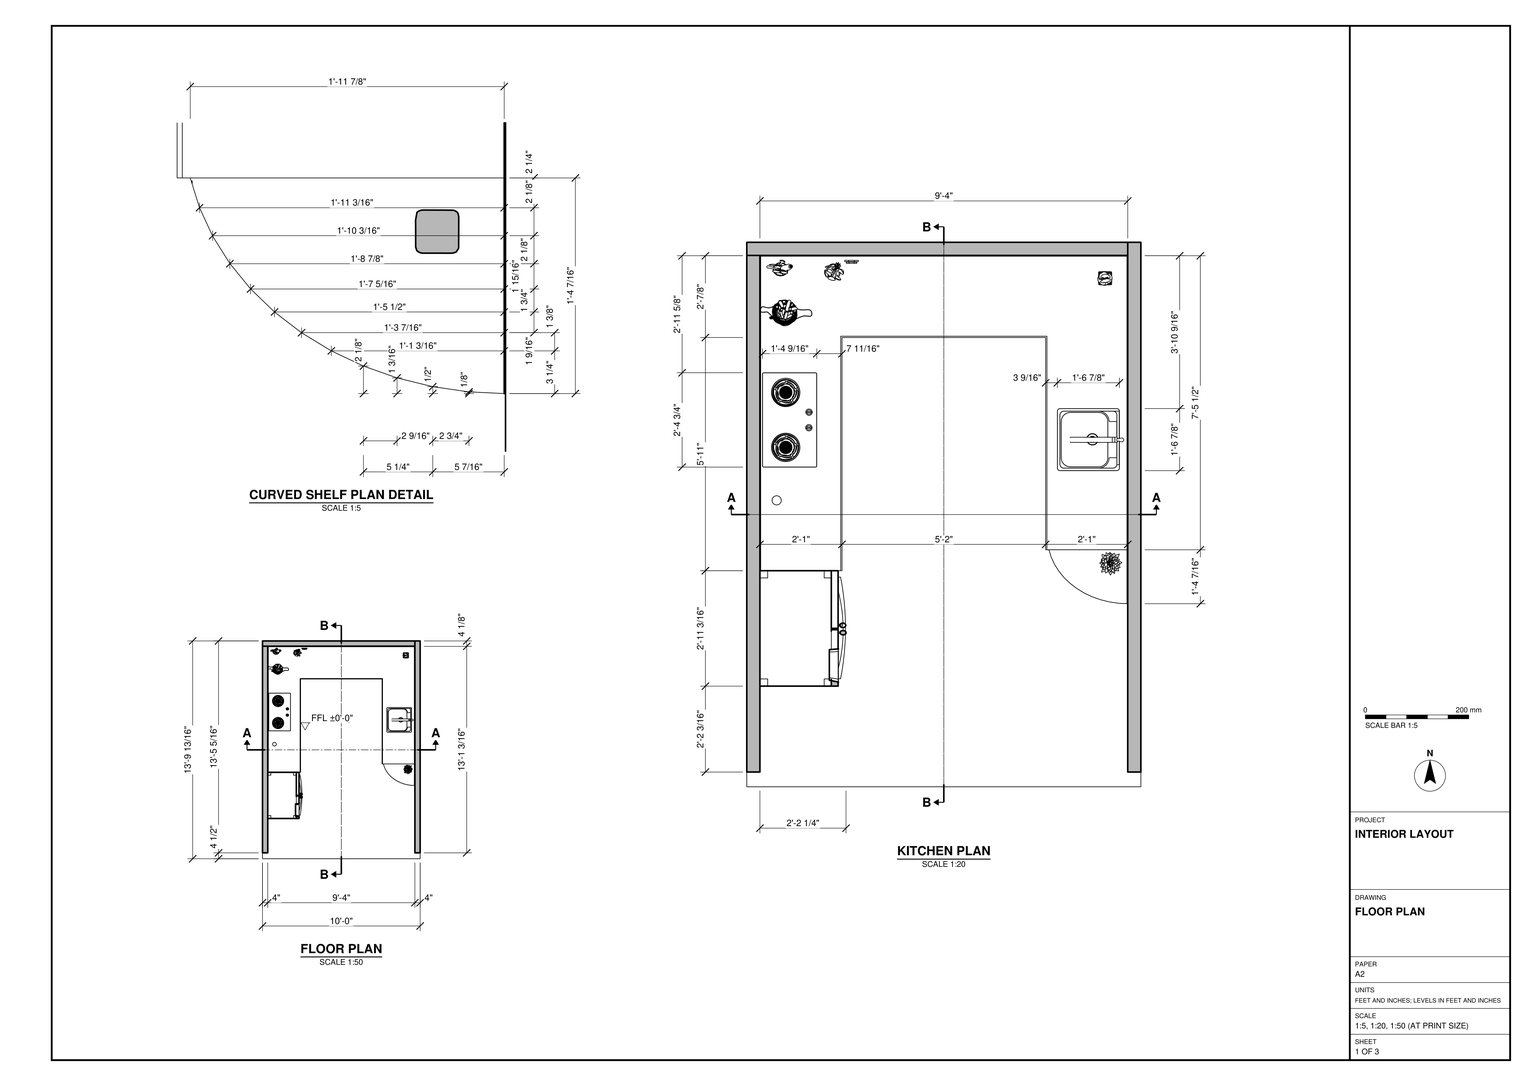
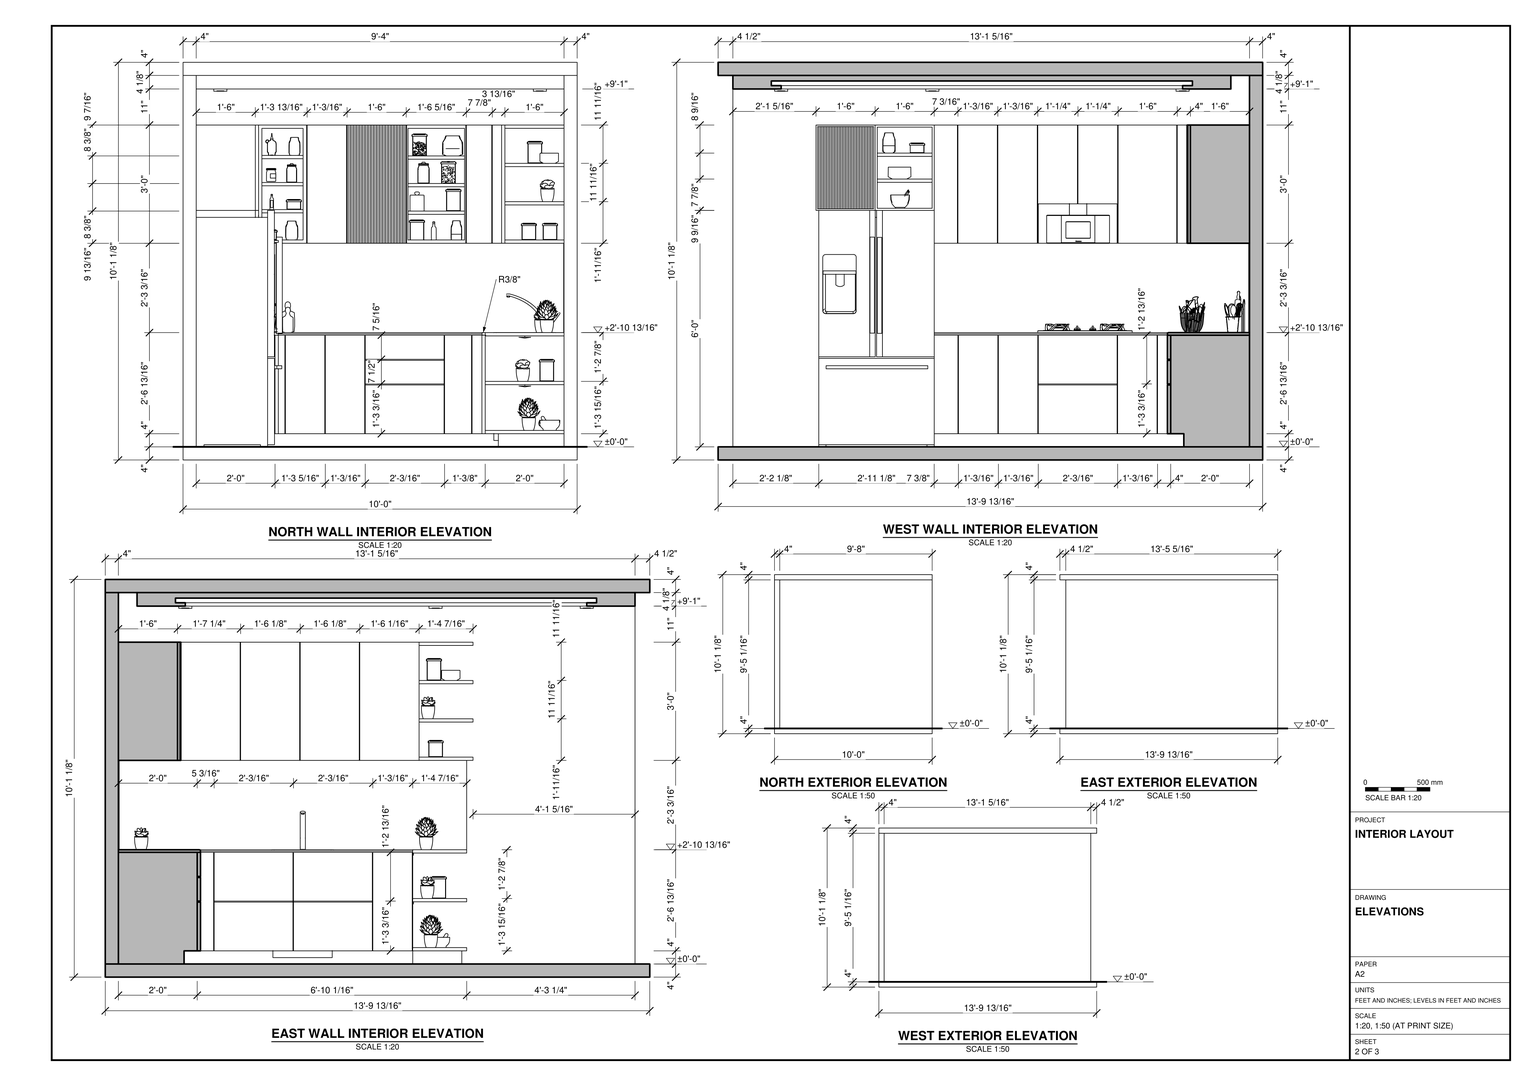
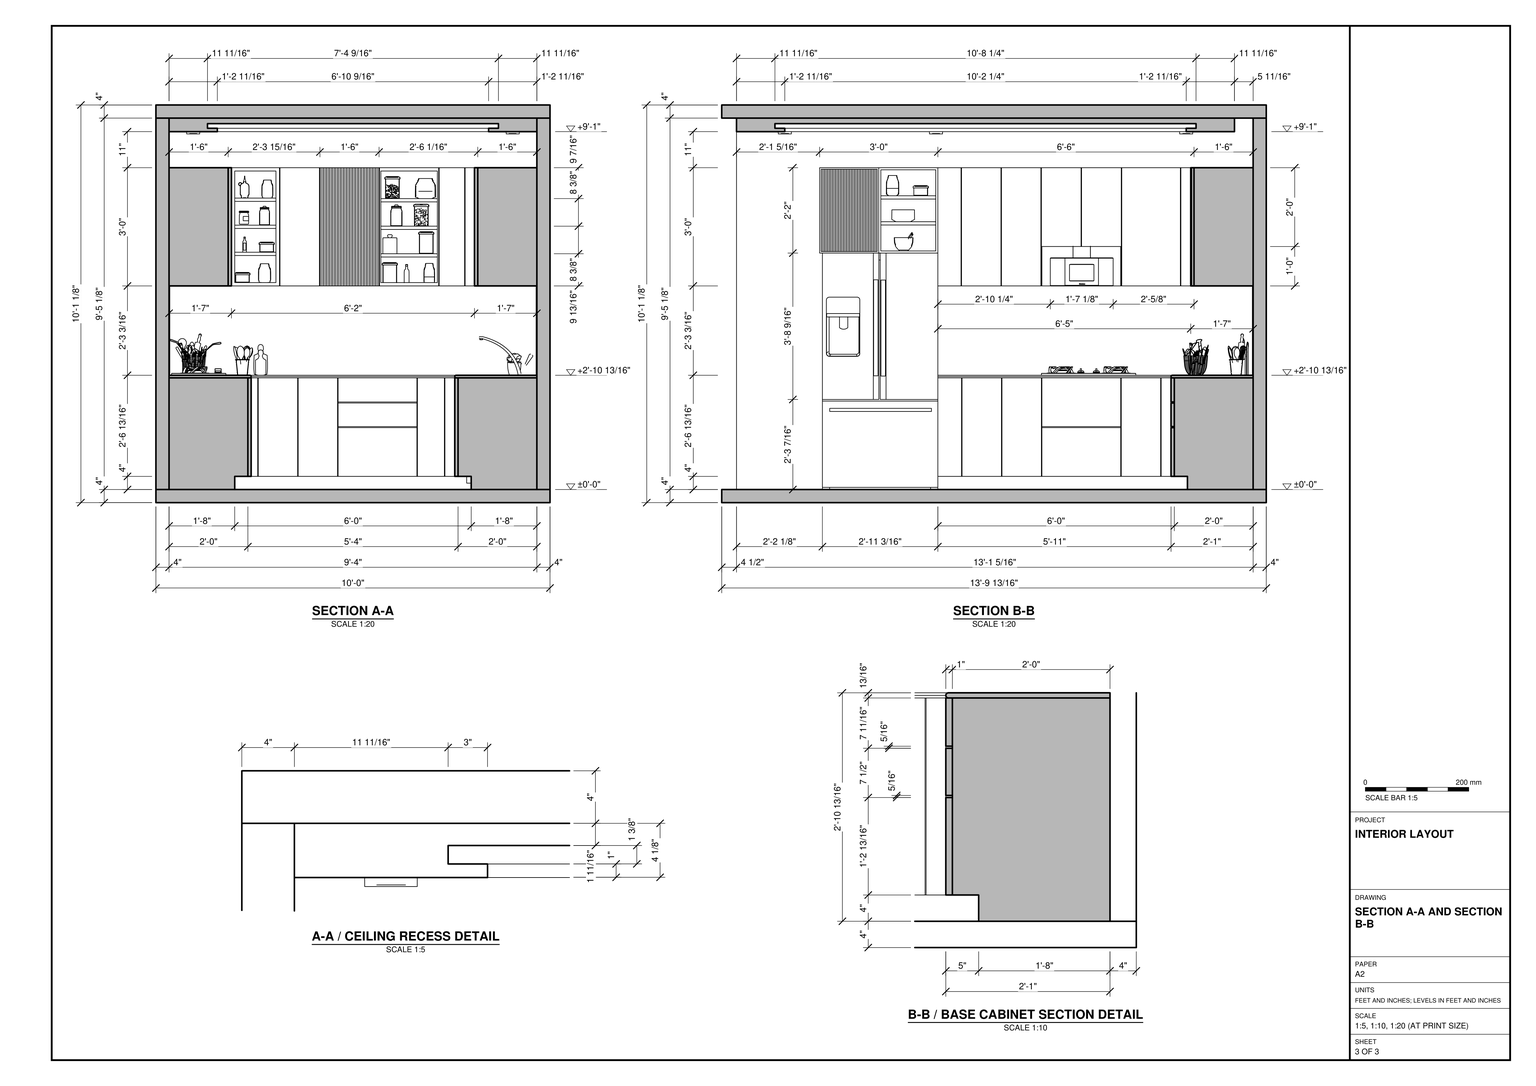
Build the kitchen interior in SketchUp from task_files/diagram_01.pdf. Work in feet and inches. Set the finished floor at ±0'-0". The overall model is 10'-0" wide, 13'-9 13/16" deep and 10'-1 1/8" high. Model the north wall and both side walls at the thicknesses shown, leaving the south end open. Include the floor slab, top slab and stepped ceiling recess shown in the sections.

Lay out the connected worktops along the west, north and east walls. Leave a 5'-2" aisle between the side runs. Place the cooktop on the west run, the refrigerator toward its open end, and the sink and tap on the east run. Follow the interior elevations for the recessed cabinet plinths, drawer banks, cupboard fronts and upper cabinets. Match the open shelf bays and vertically ribbed front on the north wall. Use the curved shelf plan detail to shape the exposed end of the east base run.

Appliances, lights, containers, utensils and plants may be any suitable library components. Keep the shell elements and each furniture or joinery piece in separate groups or components, and use components for repeated parts. Save one SketchUp model as output_files/u_shaped_kitchen_with_cabinetry_and_recessed_ceiling.skp.

# SketchUp Ruby script. Lengths in inches.
U = 1.inch
M = Sketchup.active_model
def pt(a) = Geom::Point3d.new(a.map { |v| v * U })
def face(e, loops, mat)
  f = e.add_face(loops[0].map { |a| pt(a) })
  loops[1..].each { |l| e.add_face(l.map { |a| pt(a) }).erase! }
  f.material = f.back_material = mat if mat
  f
end
# faces: each face lists its corners as indices into pts; further lists are holes
def faces(e, pts, list, mat = nil) = list.each { |f| face(e, (f[0].is_a?(Array) ? f : [f]).map { |l| l.map { |i| pts[i] } }, mat) }
# xy, xz, yz: faces in a plane at the given z, y or x. An outline is a flat list of corners, or four numbers for a rectangle; further outlines are holes
def ring(l) = l.size == 4 ? [[l[0], l[1]], [l[2], l[1]], [l[2], l[3]], [l[0], l[3]]] : l.each_slice(2).to_a
def flat(e, list, mat, &to3) = list.each { |f| face(e, (f[0].is_a?(Array) ? f : [f]).map { |l| ring(l).map { |u, v| to3.(u, v) } }, mat) }
def xy(e, z, list, mat = nil) = flat(e, list, mat) { |x, y| [x, y, z] }
def xz(e, y, list, mat = nil) = flat(e, list, mat) { |x, z| [x, y, z] }
def yz(e, x, list, mat = nil) = flat(e, list, mat) { |y, z| [x, y, z] }
def lines(e, pts, list) = list.each { |a, b| e.add_line(pt(pts[a]), pt(pts[b])) }
# prism: a flat outline (further loops are holes) pulled along v
def prism(e, loops, v, mat = nil)
  f = face(e, loops, mat); d = Geom::Vector3d.new(v.map { |x| x * U })
  f.pushpull(f.normal.samedirection?(d) ? d.length : -d.length)
end
def box(e, o, s, mat = nil) = prism(e, [[o, [o[0] + s[0], o[1], o[2]], [o[0] + s[0], o[1] + s[1], o[2]], [o[0], o[1] + s[1], o[2]]]], [0, 0, s[2]], mat)
def at(x, y, z, deg = 0) = Geom::Transformation.translation(pt([x, y, z])) * Geom::Transformation.rotation(ORIGIN, Z_AXIS, deg.degrees)
def axes(o, x, y, z) = Geom::Transformation.new([*x, 0, *y, 0, *z, 0, *pt(o).to_a, 1])
def part(name) = M.definitions.add(name)
# library, detail: a bought-in or finely detailed component or shape, given as its bounding box
def library(name, o, s) = part(name).tap { |d| box(d.entities, o, s) }
def detail(e, o, s) = box(e.add_group.entities, o, s)
def put(e, d, t, mat = nil) = e.add_instance(d, t).tap { |i| i.material = mat if mat }
def group(e, t, mat = nil) = e.add_group.tap { |g| g.transformation = t; g.material = mat if mat }.entities
root = M.entities
M.materials.add("Cl-3460 22.24cm").color = [255, 255, 255]
M.materials.add("Emissive").color = [255, 201, 138]
M.materials.add("Marble 005 36.41cm").color = [198, 200, 178]
M.materials.add("Marble Grey 23.82cm").color = [255, 255, 255]
M.materials.add("Marble Wood Grain 37.51cm").color = [255, 255, 255]
M.materials.add("VIdro preto coifa").color = [0, 0, 0]
M.materials["VIdro preto coifa"].alpha = 0.95
M.materials.add("Wood 021 27.52cm").color = [255, 255, 255]
M.materials.add("Wood Amboyan 13.2cm").color = [255, 255, 255]
M.materials.add("[Color M09]").color = [0, 0, 0]
M.materials.add("[Granite Dark Gray]").color = [69, 68, 68]
M.materials.add("[Stone Marble]").color = [143, 138, 136]
c1 = part("Shelf panel")
xy(c1.entities,0,[[-1.01,0,11.54,11.0625]],"Wood Amboyan 13.2cm")
xy(c1.entities,1,[[-1.01,0,11.54,11.0625]],"Wood Amboyan 13.2cm")
xz(c1.entities,0,[[-1.01,0,11.54,1]],"Wood Amboyan 13.2cm")
xz(c1.entities,11.0625,[[-1.01,0,11.54,1]])
yz(c1.entities,-1.01,[[0,0,11.0625,1]])
yz(c1.entities,11.54,[[0,0,11.0625,1]])
c2 = library("Fluted panel",[0,-0.1875,0],[18,0.1875,36])
c3 = part("Vertical slat")
box(c3.entities,[0,0,0],[1,0.39,25.06],"Cl-3460 22.24cm")
c4 = part("Group30\#1")
p = [[0,0,0],[0,0,-2.85],[-1.37,0,-2.85],[8.93,-0.3,0],[-8.93,-0.3,0],[8.93,0.3,0],
  [8.93,0,0],[-8.93,0.3,0],[1.37,0,-2.85],[-8.93,0,0],[0,0,-4.62]]
lines(c4.entities,p,[[0,1],[1,2],[3,4],[5,6],[7,5],[1,8],[9,0],[0,6],[8,10],[4,9],[6,3],[2,10],
  [9,7]])
c5 = part("Rectangle Light\#2")
put(c5.entities,c4,at(0,0,0))
c6 = part("Group32\#1")
p = [[0,0,0],[0,0,-2.83],[-1.375,0,-2.83],[8.95,-0.21,0],[-8.95,-0.21,0],[8.95,0.21,0],
  [8.95,0,0],[-8.95,0.21,0],[1.375,0,-2.83],[-8.95,0,0],[0,0,-4.58]]
lines(c6.entities,p,[[0,1],[1,2],[3,4],[5,6],[7,5],[1,8],[9,0],[0,6],[8,10],[4,9],[6,3],[2,10],
  [9,7]])
c7 = part("Rectangle Light\#3")
put(c7.entities,c6,at(0,0,0))
c8 = part("Group34\#1")
p = [[0,0,0],[0,0,-2.82],[-1.375,0,-2.82],[8.96,-0.18,0],[-8.96,-0.18,0],[8.96,0.18,0],
  [8.96,0,0],[-8.96,0.18,0],[1.375,0,-2.82],[-8.96,0,0],[0,0,-4.57]]
lines(c8.entities,p,[[0,1],[1,2],[3,4],[5,6],[7,5],[1,8],[9,0],[0,6],[8,10],[4,9],[6,3],[2,10],
  [9,7]])
c9 = part("Rectangle Light\#4")
put(c9.entities,c8,at(0,0,0))
c10 = part("Group36\#1")
p = [[0,0,0],[0,0,-2.96],[-1.32,0,-2.96],[8.6,-1,0],[-8.6,-1,0],[8.6,1,0],
  [8.6,0,0],[-8.6,1,0],[1.32,0,-2.96],[-8.6,0,0],[0,0,-4.8]]
lines(c10.entities,p,[[0,1],[1,2],[3,4],[5,6],[7,5],[1,8],[9,0],[0,6],[8,10],[4,9],[6,3],[2,10],
  [9,7]])
c11 = part("Rectangle Light\#5")
put(c11.entities,c10,at(0,0,0))
c12 = part("Group38\#1")
p = [[0,0,0],[0,0,-2.96],[-1.32,0,-2.96],[8.6,-0.97,0],[-8.6,-0.97,0],[8.6,0.97,0],
  [8.6,0,0],[-8.6,0.97,0],[1.32,0,-2.96],[-8.6,0,0],[0,0,-4.79]]
lines(c12.entities,p,[[0,1],[1,2],[3,4],[5,6],[7,5],[1,8],[9,0],[0,6],[8,10],[4,9],[6,3],[2,10],
  [9,7]])
c13 = part("Rectangle Light\#6")
put(c13.entities,c12,at(0,0,0))
c14 = part("Group40\#1")
p = [[0,0,0],[0,0,-3.02],[-1.32,0,-3.02],[8.6,-1.18,0],[-8.6,-1.18,0],[8.6,1.18,0],
  [8.6,0,0],[-8.6,1.18,0],[1.32,0,-3.02],[-8.6,0,0],[0,0,-4.89]]
lines(c14.entities,p,[[0,1],[1,2],[3,4],[5,6],[7,5],[1,8],[9,0],[0,6],[8,10],[4,9],[6,3],[2,10],
  [9,7]])
c15 = part("Rectangle Light\#7")
put(c15.entities,c14,at(0,0,0))
c16 = part("Group42\#1")
p = [[0,0,0],[0,0,-2.89],[-1.32,0,-2.89],[8.6,-0.76,0],[-8.6,-0.76,0],[8.6,0.76,0],
  [8.6,0,0],[-8.6,0.76,0],[1.32,0,-2.89],[-8.6,0,0],[0,0,-4.68]]
lines(c16.entities,p,[[0,1],[1,2],[3,4],[5,6],[7,5],[1,8],[9,0],[0,6],[8,10],[4,9],[6,3],[2,10],
  [9,7]])
c17 = part("Rectangle Light\#8")
put(c17.entities,c16,at(0,0,0))
c18 = part("Group44\#1")
p = [[0,0,0],[0,0,-2.23],[-0.96,0,-2.23],[6.28,-0.9375,0],[-6.28,-0.9375,0],[6.28,0.9375,0],
  [6.28,0,0],[-6.28,0.9375,0],[0.96,0,-2.23],[-6.28,0,0],[0,0,-3.61]]
lines(c18.entities,p,[[0,1],[1,2],[3,4],[5,6],[7,5],[1,8],[9,0],[0,6],[8,10],[4,9],[6,3],[2,10],
  [9,7]])
c19 = part("Rectangle Light\#9")
put(c19.entities,c18,at(0,0,0))
c20 = part("Group46\#1")
p = [[0,0,0],[0,0,-2.1],[-0.96,0,-2.1],[6.28,-0.54,0],[-6.28,-0.54,0],[6.28,0.54,0],
  [6.28,0,0],[-6.28,0.54,0],[0.96,0,-2.1],[-6.28,0,0],[0,0,-3.41]]
lines(c20.entities,p,[[0,1],[1,2],[3,4],[5,6],[7,5],[1,8],[9,0],[0,6],[8,10],[4,9],[6,3],[2,10],
  [9,7]])
c21 = part("Rectangle Light\#10")
put(c21.entities,c20,at(0,0,0))
c22 = part("Group48\#1")
p = [[0,0,0],[0,0,-2.11],[-0.96,0,-2.11],[6.28,-0.54,0],[-6.28,-0.54,0],[6.28,0.54,0],
  [6.28,0,0],[-6.28,0.54,0],[0.96,0,-2.11],[-6.28,0,0],[0,0,-3.41]]
lines(c22.entities,p,[[0,1],[1,2],[3,4],[5,6],[7,5],[1,8],[9,0],[0,6],[8,10],[4,9],[6,3],[2,10],
  [9,7]])
c23 = part("Rectangle Light\#11")
put(c23.entities,c22,at(0,0,0))
c24 = part("Group50\#1")
p = [[0,0,0],[0,0,-2.125],[-0.96,0,-2.125],[6.28,-0.6,0],[-6.28,-0.6,0],[6.28,0.6,0],
  [6.28,0,0],[-6.28,0.6,0],[0.96,0,-2.125],[-6.28,0,0],[0,0,-3.4375]]
lines(c24.entities,p,[[0,1],[1,2],[3,4],[5,6],[7,5],[1,8],[9,0],[0,6],[8,10],[4,9],[6,3],[2,10],
  [9,7]])
c25 = part("Rectangle Light\#12")
put(c25.entities,c24,at(0,0,0))
c26 = part("Group52\#1")
p = [[0,0,0],[0,0,-2.98],[-0.2,0,-2.98],[1.28,-8.36,0],[-1.28,-8.36,0],[1.28,8.36,0],
  [1.28,0,0],[-1.28,8.36,0],[0.2,0,-2.98],[-1.28,0,0],[0,0,-4.82]]
lines(c26.entities,p,[[0,1],[1,2],[3,4],[5,6],[7,5],[1,8],[9,0],[0,6],[8,10],[4,9],[6,3],[2,10],
  [9,7]])
c27 = part("Rectangle Light\#13")
put(c27.entities,c26,at(0,0,0))
c28 = part("Group54\#1")
p = [[0,0,0],[0,0,-2.93],[-0.17,0,-2.93],[1.13,-8.36,0],[-1.13,-8.36,0],[1.13,8.36,0],
  [1.13,0,0],[-1.13,8.36,0],[0.17,0,-2.93],[-1.13,0,0],[0,0,-4.75]]
lines(c28.entities,p,[[0,1],[1,2],[3,4],[5,6],[7,5],[1,8],[9,0],[0,6],[8,10],[4,9],[6,3],[2,10],
  [9,7]])
c29 = part("Rectangle Light\#14")
put(c29.entities,c28,at(0,0,0))
c30 = part("Group56\#1")
p = [[0,0,0],[0,0,-3.14],[-0.28,0,-3.14],[1.8125,-8.36,0],[-1.8125,-8.36,0],[1.8125,8.36,0],
  [1.8125,0,0],[-1.8125,8.36,0],[0.28,0,-3.14],[-1.8125,0,0],[0,0,-5.09]]
lines(c30.entities,p,[[0,1],[1,2],[3,4],[5,6],[7,5],[1,8],[9,0],[0,6],[8,10],[4,9],[6,3],[2,10],
  [9,7]])
c31 = part("Rectangle Light\#15")
put(c31.entities,c30,at(0,0,0))
c32 = part("Group58\#1")
p = [[0,0,0],[0,0,-17.95],[-8.6,0,-17.95],[56,-2.12,0],[-56,-2.12,0],[56,2.12,0],
  [56,0,0],[-56,2.12,0],[8.6,0,-17.95],[-56,0,0],[0,0,-29.06]]
lines(c32.entities,p,[[0,1],[1,2],[3,4],[5,6],[7,5],[1,8],[9,0],[0,6],[8,10],[4,9],[6,3],[2,10],
  [9,7]])
c33 = part("Rectangle Light\#16")
put(c33.entities,c32,at(0,0,0))
c34 = part("Group60\#1")
p = [[0,0,0],[0,0,-16.4],[-7.9,0,-16.4],[51.4,-1.7,0],[-51.4,-1.7,0],[51.4,1.7,0],
  [51.4,0,0],[-51.4,1.7,0],[7.9,0,-16.4],[-51.4,0,0],[0,0,-26.55]]
lines(c34.entities,p,[[0,1],[1,2],[3,4],[5,6],[7,5],[1,8],[9,0],[0,6],[8,10],[4,9],[6,3],[2,10],
  [9,7]])
c35 = part("Rectangle Light\#17")
put(c35.entities,c34,at(0,0,0))
c36 = library("double+fridge",[0,-4.28,0],[46.86,25.01,91.52])
c37 = library("GasStove_Black",[0,0,0],[28.74,16.54,2.72])
c38 = library("Potted Plant 50-23",[-3.4,-3.5,0],[6.8,7,9.93])
c39 = library("Potted Plant 50-24",[-2.18,-2.1,0],[4.36,4.2,6.7])
c40 = library("Kitchen Utensils 65-03",[-2.9,-2.77,0],[5.8,5.52,8.99])
c41 = library("Glass Vessel 001",[-1.95,-1.95,0.02],[3.9,3.9,7.26])
c42 = library("Decorative Jar 003",[-3.57,-2.61,0],[6.18,5.25,12.92])
c43 = library("Candy Jar 134 007 02",[-2.34,-2.34,0],[4.68,4.68,6.72])
c44 = library("Candy Jar 134 007 01",[-2.34,-2.34,0],[4.68,4.68,6.72])
c45 = library("Jar 83-03",[-2.15,-2.09,0],[4.3,4.18,5.88])
c46 = library("Sink and faucet",[-0.11,0,0],[20.3,18.9,21.51])
c47 = library("Kitchen Utensils 02 92-03",[-2.09,-0.47,0],[4.18,0.94,9.4])
c48 = library("Kitchen Utensils 01 92-03",[-3.91,-2.44,0],[7.79,4.85,12.66])
c49 = library("Group\#6",[0,0,0],[64,72,30])
c50 = part("Group\#49")
box(c50.entities,[0,0,0],[17.2,11.0625,1])
c51 = library("Group\#8",[0,0,0],[76,78,36])
c52 = part("Group\#20")
prism(c52.entities,[[[20,16.42,0],[20,0,0],[17.67,0.13,0],[15.37,0.53,0],[13.13,1.19,0],[10.98,2.1,0],[8.95,3.25,0],[7.0625,4.63,0],[5.35,6.21,0],[3.82,7.98,0],[2.51,9.91,0],[1.42,11.98,0],[0.59,14.16,0],[0,16.42,0]]],[0,0,1])
c53 = part("Group22\#1")
p = [[0,0,0],[0,0,-3.76],[-1.83,0,-3.76],[11.93,-0.24,0],[-11.93,-0.24,0],[11.93,0.24,0],
  [11.93,0,0],[-11.93,0.24,0],[1.83,0,-3.76],[-11.93,0,0],[0,0,-6.08]]
lines(c53.entities,p,[[0,1],[1,2],[3,4],[5,6],[7,5],[1,8],[9,0],[0,6],[8,10],[4,9],[6,3],[2,10],
  [9,7]])
c54 = part("Rectangle Light")
put(c54.entities,c53,at(0,0,0))
c55 = part("Group25\#1")
p = [[0,0,0],[0,0,-3.75],[-1.83,0,-3.75],[11.94,-0.21,0],[-11.94,-0.21,0],[11.94,0.21,0],
  [11.94,0,0],[-11.94,0.21,0],[1.83,0,-3.75],[-11.94,0,0],[0,0,-6.07]]
lines(c55.entities,p,[[0,1],[1,2],[3,4],[5,6],[7,5],[1,8],[9,0],[0,6],[8,10],[4,9],[6,3],[2,10],
  [9,7]])
c56 = part("Rectangle Light\#1")
put(c56.entities,c55,at(0,0,0))
c57 = library("Group\#12",[0,0,0],[112,96,0.79])
c58 = part("Group\#15")
box(c58.entities,[0,0,0],[13.375,16.72,1])
c59 = library("Agrupar\#3",[39.37,0,0],[35.43,16.85,31.3])
c60 = library("Group\#31",[0,0,0],[15.74,7.89,10.97])
c61 = library("Group\#32",[0,0,0],[4.68,4.68,6.72])
c62 = library("Group\#33",[0,0,0],[4.67,4.67,5.12])
c63 = library("Group\#34",[0,0,0],[4.68,4.68,3.1])
c64 = library("Group\#48",[0,0,0],[4.68,4.68,3.1])
c65 = library("Group\#35",[0,0,0],[4.68,4.68,6.72])
c66 = library("Group\#36",[0,0,0],[6.49,6.49,4.31])
c67 = library("Group\#37",[0,0,0],[2.64,2.64,11.07])
c68 = library("Group\#38",[0,0,0],[2.92,2.97,3.98])
c69 = library("Group\#39",[0,0,0],[2.6,2.61,11.08])
c70 = library("Group\#40",[0,0,0],[9.62,9.74,9.54])
c71 = library("Group\#41",[0,0,0],[7.36,7.36,7.28])
c72 = library("Group\#42",[0,0,0],[7.36,7.36,11.27])
c73 = library("Group\#43",[0,0,0],[5.95,5.95,9.65])
c74 = library("Group\#44",[0,0,0],[6.71,6.71,13.18])
c75 = library("Group\#47",[0,0,0],[5.95,5.95,9.65])
c76 = library("Recessed downlight",[0,0,0],[4,4,0.6875])
xy(root,38.79,[[115.9,55.76,116,161.71],[4,65.8125,4.1,161.71],[4,161.71,116,161.8125]])
xy(root,65.99,[[115.9,55.76,116,161.71],[4,161.71,116,161.8125]])
xy(root,66,[[4,65.8125,4.1,161.71]])
xz(root,55.76,[[115.9,38.79,116,65.99]],"[Stone Marble]")
xz(root,65.8125,[[4,38.79,4.1,66]],"[Stone Marble]")
xz(root,161.71,[[4,38.79,4.1,65.99],[115.9,38.79,116,65.99],[4,65.99,4.1,66]])
xz(root,161.71,[[4.1,38.79,115.9,65.99]],"Marble Grey 23.82cm")
xz(root,161.8125,[[4,38.79,116,65.99]])
yz(root,4,[[161.71,38.79,161.8125,65.99]])
yz(root,4.1,[[65.8125,38.79,161.71,66]],"[Stone Marble]")
yz(root,115.9,[[55.76,38.79,161.71,65.99]],"Marble Grey 23.82cm")
yz(root,116,[[161.71,38.79,161.8125,65.99]])
put(root,c1,at(25.01,143.8125,75.26))
put(root,c1,at(25.01,143.8125,83.5))
put(root,c1,at(25.01,143.8125,91.74))
put(root,c2,at(49.94,143,66))
put(root,c3,at(22,30.28,76.47))
put(root,c3,at(22,31.11,76.47))
put(root,c3,at(22,31.95,76.47))
put(root,c3,at(22,32.78,76.47))
put(root,c3,at(22,33.62,76.47))
put(root,c3,at(22,34.45,76.47))
put(root,c3,at(22,35.28,76.47))
put(root,c3,at(22,36.12,76.47))
put(root,c3,at(22,36.95,76.47))
put(root,c3,at(22,37.79,76.47))
put(root,c3,at(22,38.62,76.47))
put(root,c3,at(22,39.45,76.47))
put(root,c3,at(22,40.29,76.47))
put(root,c3,at(22,41.12,76.47))
put(root,c3,at(22,41.96,76.47))
put(root,c3,at(22,42.79,76.47))
put(root,c3,at(22,43.625,76.47))
put(root,c3,at(22,44.46,76.47))
put(root,c3,at(22,45.29,76.47))
put(root,c3,at(22,46.125,76.47))
put(root,c3,at(22,46.96,76.47))
put(root,c5,axes([107.07,69.95,100.99],[1,0,0],[0,1,0],[0,0,0.14]))
put(root,c7,axes([107.05,70.04,89.32],[1,0,0],[0,1,0],[0,0,0.23]))
put(root,c9,axes([107.04,70.07,77.66],[1,0,0],[0,1,0],[0,0,0.19]))
put(root,c11,axes([77.1,153.88,100.98],[1,0,0],[0,-1,0],[0,0,0.21]))
put(root,c13,axes([77.1,153.9,91.58],[1,0,0],[0,-1,0],[0,0,0.18]))
put(root,c15,axes([77.1,153.7,83.18],[1,0,0],[0,-1,0],[0,0,0.18]))
put(root,c17,axes([77.1,154.11,74.79],[1,0,0],[0,-1,0],[0,0,0.22]))
put(root,c19,axes([30.28,153.9375,100.98],[1,0,0],[0,-1,0],[0,0,0.2]))
put(root,c21,axes([30.28,154.34,91.73],[1,0,0],[0,-1,0],[0,0,0.25]))
put(root,c23,axes([30.28,154.33,83.49],[1,0,0],[0,-1,0],[0,0,0.17]))
put(root,c25,axes([30.28,154.27,75.25],[1,0,0],[0,-1,0],[0,0,0.19]))
put(root,c27,axes([9.9,56.8125,101.35],[1,0,0],[0,-1,0],[0,0,0.19]))
put(root,c29,axes([9.76,56.8125,92.44],[1,0,0],[0,1,0],[0,0,0.17]))
put(root,c31,axes([10.4375,56.8125,84.54],[1,0,0],[0,1,0],[0,0,0.17]))
put(root,c33,axes([60,159.69,65.99],[1,0,0],[0,-1,0],[0,0,0.11]))
put(root,c35,axes([114.3,106.17,66],[0,-1,0],[-1,0,0],[0,0,0.06059]))
put(root,c36,axes([25.74,30.66,4],[0,0.75,0],[-1.04843,0,0],[0,0,0.78669]))
put(root,c37,at(21.32,97.34,38.67,90))
put(root,c38,at(105.31,66.51,9))
put(root,c38,at(110.84,67.95,38.79))
put(root,c39,at(103.42,67.68,23.9375))
put(root,c39,at(109.0625,154.79,38.79))
put(root,c39,at(110.91,67.46,78.67))
put(root,c40,at(26.58,156.95,38.79))
put(root,c41,axes([73.22,146.92,84.2],[0.89,0,0],[0,0.89,0],[0,0,0.89]))
put(root,c41,axes([33.07,147.84,84.5],[0.79,0,0],[0,0.79,0],[0,0,0.79]))
put(root,c42,axes([27.02,145.43,92.75],[0.52,0,0],[0,0.52,0],[0,0,0.52]))
put(root,c43,at(72.01,151.24,92.59))
put(root,c44,at(80.8,147.93,84.19))
put(root,c45,at(71.25,148.48,75.75))
put(root,c46,at(114.77,115.17,29.05,180))
put(root,c47,at(31.89,159.85,38.79))
put(root,c48,at(10,157.99,38.79))
g1 = group(root,at(0,45.8125,0))
xy(g1,0,[[0,-45.8125,120,120]])
xy(g1,4,[[0,-45.8125,120,120]],"Marble 005 36.41cm")
xz(g1,-45.8125,[[0,0,120,4]])
xz(g1,120,[[0,0,120,4]])
yz(g1,0,[[-45.8125,0,120,4]])
yz(g1,120,[[-45.8125,0,120,4]])
g2 = group(root,at(116,45.8125,4))
box(g2,[0,-41.3125,0],[4,161.3125,113.1])
g3 = group(root,at(0,161.8125,4))
box(g3,[0,0,0],[116,4,113.1])
g4 = group(root,at(0,45.8125,4))
box(g4,[0,-41.3125,0],[4,157.3125,113.1])
g5 = group(root,at(4,65.8125,4))
xy(g5,0,[[0,0,0,96,112,96,112,6.37,92,6.37,92,76,20,76,20,0]])
xy(g5,1.9375,[[90.63,30.89,107.24,48.95]])
xy(g5,4,[[20,0,24,76],[88,6.37,92,72],[24,72,92,76]])
xy(g5,34,[[[0,0,24,0,24,72,88,72,88,6.37,112,6.37,112,96,0,96],[90.63,30.89,107.24,48.95]]])
xz(g5,0,[[0,0,20,0,20,4,24,4,24,34,0,34]])
xz(g5,6.37,[[92,0,112,0,112,34,88,34,88,4,92,4]])
xz(g5,30.89,[[90.63,1.9375,107.24,34]])
xz(g5,48.95,[[90.63,1.9375,107.24,34]])
xz(g5,72,[[24,4,88,34]])
xz(g5,76,[[20,0,92,4]],"Wood 021 27.52cm")
xz(g5,96,[[0,0,112,34]])
yz(g5,0,[[0,0,96,34]])
yz(g5,20,[[0,0,76,4]],"Wood 021 27.52cm")
yz(g5,24,[[0,4,72,34]])
yz(g5,88,[[6.37,4,72,34]])
yz(g5,90.63,[[30.89,1.9375,48.95,34]])
yz(g5,92,[[6.37,0,76,4]],"Wood 021 27.52cm")
yz(g5,107.24,[[30.89,1.9375,48.95,34]])
yz(g5,112,[[6.37,0,96,34]])
put(root,c49,at(28,65.8125,8),"Cl-3460 22.24cm")
g6 = group(root,at(4,65.8125,66))
xy(g6,0,[[0,0,18,31.69],[94,4.4375,94,78,18,78,18,55.69,0,55.69,0,96,112,96,112,4.4375]])
xy(g6,0.4,[[64.5,78,81.7,89.0625]])
xy(g6,1.01,[[20,78,32.55,89.0625]])
xy(g6,12,[[0,31.69,18,55.69]])
xy(g6,34.99,[[20,78,32.55,89.0625],[64.5,78,81.7,89.0625]])
xy(g6,36,[[0,0,18,0,18,78,94,78,94,4.4375,112,4.4375,112,96,0,96]])
xz(g6,0,[[0,0,18,36]])
xz(g6,4.4375,[[94,0,112,36]])
xz(g6,31.69,[[0,0,18,12]])
xz(g6,55.69,[[0,0,18,12]])
xz(g6,78,[[[18,0,94,36],[64.5,0.4,81.7,34.99],[20,1.01,32.55,34.99]]])
xz(g6,89.0625,[[64.5,0.4,81.7,34.99],[20,1.01,32.55,34.99]])
yz(g6,0,[[31.69,0,55.69,12]])
yz(g6,18,[[0,0,31.69,0,31.69,12,55.69,12,55.69,0,78,0,78,36,0,36]])
yz(g6,20,[[78,1.01,89.0625,34.99]])
yz(g6,32.55,[[78,1.01,89.0625,34.99]])
yz(g6,64.5,[[78,0.4,89.0625,34.99]])
yz(g6,81.7,[[78,0.4,89.0625,34.99]])
yz(g6,94,[[4.4375,0,78,36]])
yz(g6,112,[[4.4375,0,96,36]])
put(root,c50,at(68.5,143.8125,74.8),"Wood Amboyan 13.2cm")
put(root,c50,at(68.5,143.8125,83.19),"Wood Amboyan 13.2cm")
g7 = group(root,at(68.5,143.8125,91.59),"Wood Amboyan 13.2cm")
box(g7,[0,0,0],[17.2,11.0625,1])
put(root,c51,at(22,65.8125,66),"Cl-3460 22.24cm")
g8 = group(root,at(94.1,55.9,4),"[Color M09]")
prism(g8,[[[21.9,16.28,0],[21.9,1.34,0],[19.61,1.5625,0],[17.36,2,0],[15.17,2.65,0],[13.0625,3.51,0],[11.07,4.57,0],[9.21,5.8125,0],[7.51,7.23,0],[5.98,8.8,0],[4.64,10.51,0],[3.51,12.34,0],[2.59,14.27,0],[1.9,16.28,0]]],[0,0,4])
put(root,c52,axes([92,55.76,8],[1.2,0,0],[0,1,0],[0,0,1]),"[Granite Dark Gray]")
g9 = group(root,at(92,55.76,22.9375),"[Granite Dark Gray]")
xy(g9,0,[[24,0,21.2,0.13,18.44,0.53,15.75,1.19,13.18,2.1,10.74,3.25,8.47,4.63,6.41,6.21,4.58,7.98,3.01,9.91,1.71,11.98,0.7,14.16,0.15,15.94,24,15.94],[0.15,15.94,0,16.42,24,16.42,24,15.94]])
xy(g9,1,[[24,0,24,16.42,0,16.42,0.7,14.16,1.71,11.98,3.01,9.91,4.58,7.98,6.41,6.21,8.47,4.63,10.74,3.25,13.18,2.1,15.75,1.19,18.44,0.53,21.2,0.13]])
xz(g9,16.42,[[0,0,24,1]])
yz(g9,24,[[0,0,16.42,1]])
p = [[24,0,1],[21.2,0.13,1],[21.2,0.13,0],[24,0,0],[18.44,0.53,1],[18.44,0.53,0],
  [15.75,1.19,1],[15.75,1.19,0],[13.18,2.1,1],[13.18,2.1,0],[10.74,3.25,1],[10.74,3.25,0],
  [8.47,4.63,1],[8.47,4.63,0],[6.41,6.21,1],[6.41,6.21,0],[4.58,7.98,1],[4.58,7.98,0],
  [3.01,9.91,1],[3.01,9.91,0],[1.71,11.98,1],[1.71,11.98,0],[0.7,14.16,1],[0.7,14.16,0],
  [0,16.42,1],[0,16.42,0],[0.15,15.94,0],[24.15,15.94,0],[24,15.94,0]]
faces(g9,p,[[0,1,2,3],[1,4,5,2],[4,6,7,5],[6,8,9,7],[8,10,11,9],[10,12,13,11],[12,14,15,13],[14,16,17,15],
  [16,18,19,17],[18,20,21,19],[20,22,23,21],[22,24,25,26,23]])
lines(g9,p,[[27,28]])
put(g9,c54,axes([12.07,16.18,-0.01],[1,0,0],[0,1,0],[0,0,0.11]))
g10 = group(root,at(92,55.76,37.79),"[Granite Dark Gray]")
xy(g10,0,[[24,0,21.2,0.13,18.44,0.53,15.75,1.19,13.18,2.1,10.74,3.25,8.47,4.63,6.41,6.21,4.58,7.98,3.01,9.91,1.71,11.98,0.7,14.16,0.13,16,24,16],[0.13,16,0,16.42,24,16.42,24,16]])
xy(g10,1,[[24,0,24,16.42,0,16.42,0.7,14.16,1.71,11.98,3.01,9.91,4.58,7.98,6.41,6.21,8.47,4.63,10.74,3.25,13.18,2.1,15.75,1.19,18.44,0.53,21.2,0.13]])
xz(g10,16.42,[[0,0,24,1]])
yz(g10,24,[[0,0,16.42,1]])
p = [[24,0,1],[21.2,0.13,1],[21.2,0.13,0],[24,0,0],[18.44,0.53,1],[18.44,0.53,0],
  [15.75,1.19,1],[15.75,1.19,0],[13.18,2.1,1],[13.18,2.1,0],[10.74,3.25,1],[10.74,3.25,0],
  [8.47,4.63,1],[8.47,4.63,0],[6.41,6.21,1],[6.41,6.21,0],[4.58,7.98,1],[4.58,7.98,0],
  [3.01,9.91,1],[3.01,9.91,0],[1.71,11.98,1],[1.71,11.98,0],[0.7,14.16,1],[0.7,14.16,0],
  [0,16.42,1],[0,16.42,0],[0.13,16,0],[24.13,16,0],[24,16,0]]
faces(g10,p,[[0,1,2,3],[1,4,5,2],[4,6,7,5],[6,8,9,7],[8,10,11,9],[10,12,13,11],[12,14,15,13],[14,16,17,15],
  [16,18,19,17],[18,20,21,19],[20,22,23,21],[22,24,25,26,23]])
lines(g10,p,[[27,28]])
put(g10,c56,axes([12.06,16.21,-0.01],[1,0,0],[0,1,0],[0,0,0.11]))
g11 = group(root,at(98,53.83,101),"[Granite Dark Gray]")
xy(g11,0,[[18,0,15.9,0.13,13.83,0.53,11.82,1.19,9.88,2.1,8.05,3.25,6.36,4.63,4.8125,6.21,3.4375,7.98,2.26,9.91,1.28,11.98,0.53,14.16,0.14,15.81,18,15.81],[0.14,15.81,0,16.42,18,16.42,18,15.81]])
xy(g11,1,[[18,0,18,16.42,0,16.42,0.53,14.16,1.28,11.98,2.26,9.91,3.4375,7.98,4.8125,6.21,6.36,4.63,8.05,3.25,9.88,2.1,11.82,1.19,13.83,0.53,15.9,0.13]])
xz(g11,16.42,[[0,0,18,1]])
yz(g11,18,[[0,0,16.42,1]])
p = [[18,0,1],[15.9,0.13,1],[15.9,0.13,0],[18,0,0],[13.83,0.53,1],[13.83,0.53,0],
  [11.82,1.19,1],[11.82,1.19,0],[9.88,2.1,1],[9.88,2.1,0],[8.05,3.25,1],[8.05,3.25,0],
  [6.36,4.63,1],[6.36,4.63,0],[4.8125,6.21,1],[4.8125,6.21,0],[3.4375,7.98,1],[3.4375,7.98,0],
  [2.26,9.91,1],[2.26,9.91,0],[1.28,11.98,1],[1.28,11.98,0],[0.53,14.16,1],[0.53,14.16,0],
  [0,16.42,1],[0,16.42,0],[0.14,15.81,0],[18.14,15.81,0],[18,15.81,0]]
faces(g11,p,[[0,1,2,3],[1,4,5,2],[4,6,7,5],[6,8,9,7],[8,10,11,9],[10,12,13,11],[12,14,15,13],[14,16,17,15],
  [16,18,19,17],[18,20,21,19],[20,22,23,21],[22,24,25,26,23]])
lines(g11,p,[[27,28]])
g12 = group(root,at(98,53.83,89.33),"[Granite Dark Gray]")
xy(g12,0,[[18,0,15.9,0.13,13.83,0.53,11.82,1.19,9.88,2.1,8.05,3.25,6.36,4.63,4.8125,6.21,3.4375,7.98,2.26,9.91,1.28,11.98,0.53,14.16,0.1,15.99,18,15.99],[0.1,15.99,0,16.42,18,16.42,18,15.99]])
xy(g12,1,[[18,0,18,16.42,0,16.42,0.53,14.16,1.28,11.98,2.26,9.91,3.4375,7.98,4.8125,6.21,6.36,4.63,8.05,3.25,9.88,2.1,11.82,1.19,13.83,0.53,15.9,0.13]])
xz(g12,16.42,[[0,0,18,1]])
yz(g12,18,[[0,0,16.42,1]])
p = [[18,0,1],[15.9,0.13,1],[15.9,0.13,0],[18,0,0],[13.83,0.53,1],[13.83,0.53,0],
  [11.82,1.19,1],[11.82,1.19,0],[9.88,2.1,1],[9.88,2.1,0],[8.05,3.25,1],[8.05,3.25,0],
  [6.36,4.63,1],[6.36,4.63,0],[4.8125,6.21,1],[4.8125,6.21,0],[3.4375,7.98,1],[3.4375,7.98,0],
  [2.26,9.91,1],[2.26,9.91,0],[1.28,11.98,1],[1.28,11.98,0],[0.53,14.16,1],[0.53,14.16,0],
  [0,16.42,1],[0,16.42,0],[0.1,15.99,0],[18.1,15.99,0],[18,15.99,0]]
faces(g12,p,[[0,1,2,3],[1,4,5,2],[4,6,7,5],[6,8,9,7],[8,10,11,9],[10,12,13,11],[12,14,15,13],[14,16,17,15],
  [16,18,19,17],[18,20,21,19],[20,22,23,21],[22,24,25,26,23]])
lines(g12,p,[[27,28]])
g13 = group(root,at(98,53.83,77.67),"[Granite Dark Gray]")
xy(g13,0,[[18,0,15.9,0.13,13.83,0.53,11.82,1.19,9.88,2.1,8.05,3.25,6.36,4.63,4.8125,6.21,3.4375,7.98,2.26,9.91,1.28,11.98,0.53,14.16,0.09,16.05,18,16.05],[0.09,16.05,0,16.42,18,16.42,18,16.05]])
xy(g13,1,[[18,0,18,16.42,0,16.42,0.53,14.16,1.28,11.98,2.26,9.91,3.4375,7.98,4.8125,6.21,6.36,4.63,8.05,3.25,9.88,2.1,11.82,1.19,13.83,0.53,15.9,0.13]])
xz(g13,16.42,[[0,0,18,1]])
yz(g13,18,[[0,0,16.42,1]])
p = [[18,0,1],[15.9,0.13,1],[15.9,0.13,0],[18,0,0],[13.83,0.53,1],[13.83,0.53,0],
  [11.82,1.19,1],[11.82,1.19,0],[9.88,2.1,1],[9.88,2.1,0],[8.05,3.25,1],[8.05,3.25,0],
  [6.36,4.63,1],[6.36,4.63,0],[4.8125,6.21,1],[4.8125,6.21,0],[3.4375,7.98,1],[3.4375,7.98,0],
  [2.26,9.91,1],[2.26,9.91,0],[1.28,11.98,1],[1.28,11.98,0],[0.53,14.16,1],[0.53,14.16,0],
  [0,16.42,1],[0,16.42,0],[0.09,16.05,0],[18.09,16.05,0],[18,16.05,0]]
faces(g13,p,[[0,1,2,3],[1,4,5,2],[4,6,7,5],[6,8,9,7],[8,10,11,9],[10,12,13,11],[12,14,15,13],[14,16,17,15],
  [16,18,19,17],[18,20,21,19],[20,22,23,21],[22,24,25,26,23]])
lines(g13,p,[[27,28]])
put(root,c52,axes([98,53.83,66],[0.9,0,0],[0,1,0],[0,0,1]),"[Granite Dark Gray]")
put(root,c57,at(4,65.8125,38),"Marble Wood Grain 37.51cm")
g14 = group(root,at(4,29.8125,76),"Cl-3460 22.24cm")
xy(g14,0,[[0,0,18,36]])
xy(g14,0.64,[[4.625,18.64,18,35.36]])
xy(g14,25.36,[[4.625,18.64,18,35.36]])
xy(g14,26,[[0,0,18,36]])
xz(g14,0,[[0,0,18,26]])
xz(g14,18.64,[[4.625,0.64,18,25.36]])
xz(g14,35.36,[[4.625,0.64,18,25.36]])
xz(g14,36,[[0,0,18,26]])
yz(g14,0,[[0,0,36,26]])
yz(g14,4.625,[[18.64,0.64,35.36,25.36]])
yz(g14,18,[[[0,0,36,26],[18.64,0.64,35.36,25.36]]])
g15 = group(root,at(22,29.8125,76),"Cl-3460 22.24cm")
xy(g15,0,[[0,0,1,36]])
xy(g15,0.47,[[0,0.47,1,17.53]])
xy(g15,0.64,[[0,18.64,1,35.36]])
xy(g15,25.36,[[0,18.64,1,35.36]])
xy(g15,25.53,[[0,0.47,1,17.53]])
xy(g15,26,[[0,0,1,36]])
xz(g15,0,[[0,0,1,26]])
xz(g15,0.47,[[0,0.47,1,25.53]])
xz(g15,17.53,[[0,0.47,1,25.53]])
xz(g15,18.64,[[0,0.64,1,25.36]])
xz(g15,35.36,[[0,0.64,1,25.36]])
xz(g15,36,[[0,0,1,26]])
yz(g15,0,[[[0,0,36,26],[0.47,0.47,17.53,25.53],[18.64,0.64,35.36,25.36]]])
yz(g15,1,[[[0,0,18,26],[0.47,0.47,17.53,25.53]]])
yz(g15,1,[[[18,0,36,26],[18.64,0.64,35.36,25.36]]],"Cl-3460 22.24cm")
put(root,c58,at(8.625,48.45,84.55),"Wood Amboyan 13.2cm")
put(root,c58,at(8.625,48.45,92.45),"Wood Amboyan 13.2cm")
put(root,c59,axes([23.04,78.79,65.97],[0,0.54,0],[-0.54,0,0],[0,0,0.54]),"VIdro preto coifa")
put(root,c60,at(4.1,140.38,38.79))
put(root,c61,at(68.875,146.39,66.4))
put(root,c61,at(79.98,145.14,75.8))
put(root,c62,at(102.96,62.87,67))
put(root,c62,at(109.4,62.87,67))
put(root,c63,at(14.03,58.27,93.45))
put(root,c64,at(24,148.375,67.01))
put(root,c64,at(31.38,146.31,76.26))
put(root,c65,at(104.78,63.375,90.33))
put(root,c65,at(108.41,61.91,23.9375))
put(root,c66,at(108.25,60.92,9))
put(root,c67,axes([75.6,146.86,66.33],[0.56,0,0],[0,0.56,0],[0,0,0.56]))
put(root,c68,at(25.35,149.25,84.81))
put(root,c69,axes([26.46,147.53,76.26],[0.42,0,0],[0,0.42,0],[0,0,0.42]))
put(root,c70,axes([14.64,52.52,76.64],[0.59,0,0],[0,0.59,0],[0,0,0.59]))
put(root,c71,axes([78.98,146.68,92.59],[0.84,0,0],[0,0.84,0],[0,0,0.84]))
put(root,c72,axes([31.21,146.23,67.01],[0.51,0,0],[0,0.51,0],[0,0,0.51]))
put(root,c73,axes([32.23,146.39,92.74],[0.57,0,0],[0,0.57,0],[0,0,0.57]))
put(root,c74,axes([81.59,147.47,66.4],[0.49,0,0],[0,0.49,0],[0,0,0.49]))
g16 = group(root,at(108.7,57.79,90.33))
detail(g16,[0,0,0],[5.62,5.62,3.11])
g17 = group(root,at(15.0625,51.78,85.55))
detail(g17,[0,0,0],[6.9375,6.9375,3.63])
put(root,c75,axes([15.05,50.12,93.45],[0.64,0,0],[0,0.64,0],[0,0,0.64]))
g18 = group(root,at(0,45.8125,117.1))
xy(g18,0,[[0,-45.8125,120,120]])
xy(g18,4,[[0,-45.8125,120,120]],"Marble 005 36.41cm")
xz(g18,-45.8125,[[0,0,120,4]])
xz(g18,120,[[0,0,120,4]])
yz(g18,0,[[-45.8125,0,120,4]])
yz(g18,120,[[-45.8125,0,120,4]])
g19 = group(root,at(4,4.5,112.6))
xy(g19,0.375,[[[0,0,112,151.64],[14.7,14.7,97.3,136.93]]])
xy(g19,1.41,[[11.7,11.7,14.7,139.93],[14.7,11.7,97.3,14.7],[97.3,11.7,100.3,136.93],[14.7,136.93,100.3,139.93]],"Emissive")
xy(g19,2.8125,[[11.7,11.7,100.3,139.93]])
xy(g19,4.5,[[0,0,112,151.64]])
xz(g19,0,[[0,0.375,112,4.5]])
xz(g19,11.7,[[11.7,1.41,100.3,2.8125]])
xz(g19,14.7,[[14.7,0.375,97.3,1.41]])
xz(g19,136.93,[[14.7,0.375,97.3,1.41]])
xz(g19,139.93,[[11.7,1.41,100.3,2.8125]])
xz(g19,151.64,[[0,0.375,112,4.5]])
yz(g19,0,[[0,0.375,151.64,4.5]])
yz(g19,11.7,[[11.7,1.41,139.93,2.8125]])
yz(g19,14.7,[[14.7,0.375,136.93,1.41]])
yz(g19,97.3,[[14.7,0.375,136.93,1.41]])
yz(g19,100.3,[[11.7,1.41,139.93,2.8125]])
yz(g19,112,[[0,0.375,151.64,4.5]])
put(g19,c76,axes([106.65,12.7,0.375],[-1,0,0],[0,1,0],[0,0,-1]))
put(g19,c76,axes([9.35,12.7,0.375],[-1,0,0],[0,1,0],[0,0,-1]))
put(g19,c76,axes([106.65,134.93,0.375],[-1,0,0],[0,1,0],[0,0,-1]))
put(g19,c76,axes([9.35,134.93,0.375],[-1,0,0],[0,1,0],[0,0,-1]))
put(g19,c76,axes([106.65,58.74,0.375],[-1,0,0],[0,1,0],[0,0,-1]))
put(g19,c76,axes([9.35,58.74,0.375],[-1,0,0],[0,1,0],[0,0,-1]))
